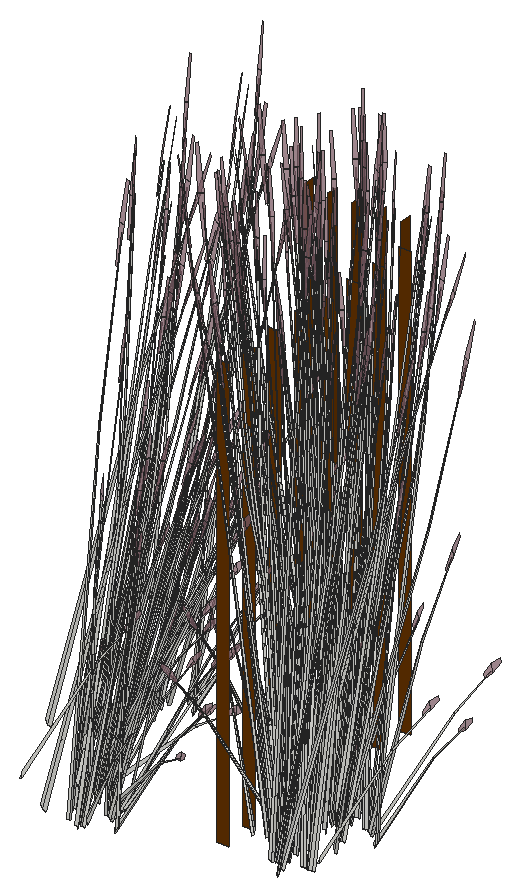
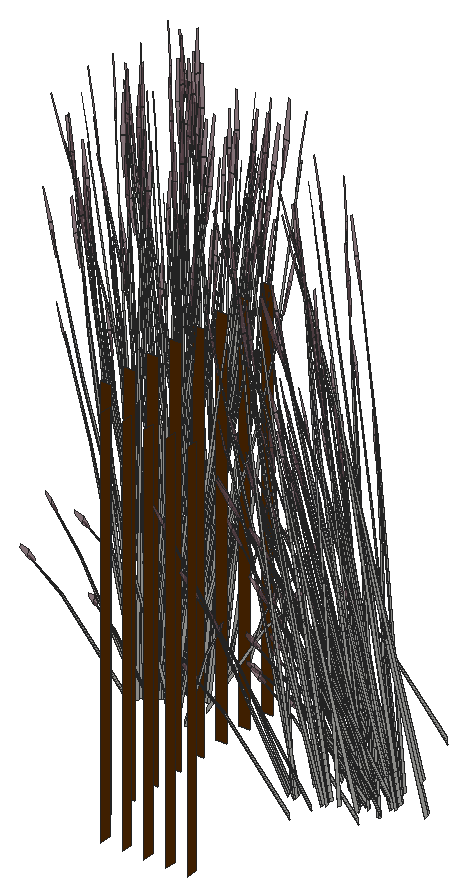
# SketchUp Ruby script. Lengths in inches.
U = 1.inch
M = Sketchup.active_model
def pt(a) = Geom::Point3d.new(a.map { |v| v * U })
def face(e, loops, mat)
  f = e.add_face(loops[0].map { |a| pt(a) })
  loops[1..].each { |l| e.add_face(l.map { |a| pt(a) }).erase! }
  f.material = f.back_material = mat if mat
  f
end
# faces: each face lists its corners as indices into pts; further lists are holes
def faces(e, pts, list, mat = nil) = list.each { |f| face(e, (f[0].is_a?(Array) ? f : [f]).map { |l| l.map { |i| pts[i] } }, mat) }
# xy, xz, yz: faces in a plane at the given z, y or x. An outline is a flat list of corners, or four numbers for a rectangle; further outlines are holes
def ring(l) = l.size == 4 ? [[l[0], l[1]], [l[2], l[1]], [l[2], l[3]], [l[0], l[3]]] : l.each_slice(2).to_a
def flat(e, list, mat, &to3) = list.each { |f| face(e, (f[0].is_a?(Array) ? f : [f]).map { |l| ring(l).map { |u, v| to3.(u, v) } }, mat) }
def xy(e, z, list, mat = nil) = flat(e, list, mat) { |x, y| [x, y, z] }
def xz(e, y, list, mat = nil) = flat(e, list, mat) { |x, z| [x, y, z] }
def yz(e, x, list, mat = nil) = flat(e, list, mat) { |y, z| [x, y, z] }
def lines(e, pts, list) = list.each { |a, b| e.add_line(pt(pts[a]), pt(pts[b])) }
# prism: a flat outline (further loops are holes) pulled along v
def prism(e, loops, v, mat = nil)
  f = face(e, loops, mat); d = Geom::Vector3d.new(v.map { |x| x * U })
  f.pushpull(f.normal.samedirection?(d) ? d.length : -d.length)
end
def box(e, o, s, mat = nil) = prism(e, [[o, [o[0] + s[0], o[1], o[2]], [o[0] + s[0], o[1] + s[1], o[2]], [o[0], o[1] + s[1], o[2]]]], [0, 0, s[2]], mat)
def at(x, y, z, deg = 0) = Geom::Transformation.translation(pt([x, y, z])) * Geom::Transformation.rotation(ORIGIN, Z_AXIS, deg.degrees)
def axes(o, x, y, z) = Geom::Transformation.new([*x, 0, *y, 0, *z, 0, *pt(o).to_a, 1])
def part(name) = M.definitions.add(name)
# library, detail: a bought-in or finely detailed component or shape, given as its bounding box
def library(name, o, s) = part(name).tap { |d| box(d.entities, o, s) }
def detail(e, o, s) = box(e.add_group.entities, o, s)
def put(e, d, t, mat = nil) = e.add_instance(d, t).tap { |i| i.material = mat if mat }
def group(e, t, mat = nil) = e.add_group.tap { |g| g.transformation = t; g.material = mat if mat }.entities
root = M.entities
M.materials.add("C08_Toffee_Ember").color = [102, 51, 0]
M.materials.add("LightPink_Translucent").color = [144, 107, 117]
M.materials["LightPink_Translucent"].alpha = 0.75
c1 = part("blade")
p = [[2.15,0.21,22],[0,0.17,0],[0.09,0.45,0],[2.18,0.31,22],[2.29,0.31,22],[0.38,0.45,0],
  [2.48,0.24,33],[2.49,0.24,33],[2.48,0.22,33]]
faces(c1.entities,p,[[0,1,2,3],[4,5,2,3],[6,3,4,7],[8,0,3,6]])
c2 = part("seeds")
p = [[0.3,-0.1,1.38],[-0.01,-0.03,1.59],[-0.01,-0.03,0.03],[0.14,-0.07,-0.07],[0.29,-0.03,3],[0.15,0.01,3.11]]
faces(c2.entities,p,[[0,1,2,3],[1,0,4,5]],"LightPink_Translucent")
c3 = part("blade with seeds")
put(c3.entities,c1,at(0,0,0))
put(c3.entities,c2,axes([2.4,0.25,30.99],[1.5799,-0.05474,1.17369],[-0.12525,1.92788,0.29478],[-0.07173,-0.02425,1.56792]))
xz(root,338.4,[[693.41,510,694.41,546]],"C08_Toffee_Ember")
xz(root,341.1,[[693.41,510,694.41,546]],"C08_Toffee_Ember")
xz(root,343.8,[[693.41,510,694.41,546]],"C08_Toffee_Ember")
xz(root,346.5,[[693.41,510,694.41,546]],"C08_Toffee_Ember")
xz(root,349.2,[[693.41,510,694.41,546]],"C08_Toffee_Ember")
xz(root,351.9,[[693.41,510,694.41,546]],"C08_Toffee_Ember")
xz(root,354.6,[[693.41,510,694.41,546]],"C08_Toffee_Ember")
xz(root,357.3,[[693.41,510,694.41,546]],"C08_Toffee_Ember")
yz(root,683.33,[[360,510,361,546]],"C08_Toffee_Ember")
yz(root,685.34,[[360,510,361,546]],"C08_Toffee_Ember")
yz(root,687.36,[[360,510,361,546]],"C08_Toffee_Ember")
yz(root,689.38,[[360,510,361,546]],"C08_Toffee_Ember")
yz(root,691.4,[[360,510,361,546]],"C08_Toffee_Ember")
put(root,c3,axes([681.33,342.92,511.97],[0.81352,0,0],[0,0.63814,-0.42834],[0,0.14534,1.3588]))
put(root,c3,axes([682.51,340.18,507.48],[0,-0.57097,0.4121],[0.72788,0,0],[0,0.13004,1.30728]))
put(root,c3,axes([678.7,342.09,512.21],[0.65687,-0.37907,-0.24149],[0.43681,0.53562,-0.41502],[0.16207,0.0544,1.32557]))
put(root,c3,axes([682.82,340.71,507.1],[0,0.57097,-0.4121],[-0.72788,0,0],[0,0.13004,1.30728]))
put(root,c3,axes([680.88,342.4375,509.35],[-0.64708,0.13103,0.39842],[-0.1123,-0.514,0.32852],[0.15218,0.15149,0.82444]))
put(root,c3,axes([680.76,342.54,509.35],[-0.29569,0.36271,0.05337],[-0.42107,-0.21117,0.42015],[0.13613,0.11629,0.64067]))
put(root,c3,axes([680.01,341.34,508.64],[-0.14872,-0.18332,1.42242],[0.6872,-0.15433,0.11501],[0.15531,0.28779,0.60807]))
put(root,c3,axes([680.44,339.28,507.6],[0.12551,-0.50956,0.12018],[0.6132,0.08845,-0.34318],[0.1116,0.05232,1.05198]))
put(root,c3,axes([680.07,348.69,511.83],[0.39083,0.47924,-0.37133],[-0.59199,0.33747,0.17871],[0.12647,0.0593,1.19224]))
put(root,c3,axes([679.34,335.47,511.24],[0.0474,-0.08243,1.46364],[0.59674,-0.24277,-0.2236],[0.18092,0.12565,0.24931]))
put(root,c3,axes([681.3125,338.39,507.48],[-0.60889,-0.28548,0.4121],[0.36394,-0.51192,0],[0.13868,0.06502,1.30728]))
put(root,c3,axes([679.87,350.69,512.15],[0.01148,-0.18927,1.18691],[0.54864,-0.21141,-0.25526],[0.16937,0.22654,0.50747]))
put(root,c3,axes([679.22,348.01,511.71],[0.43821,-0.42916,-0.51753],[0.54436,0.38915,-0.13583],[0.1756,-0.10706,1.14236]))
put(root,c3,axes([680.78,341.375,507.24],[0.68303,-0.19373,-0.15934],[0.24001,0.55805,0.00007],[0.07539,-0.02141,1.44335]))
put(root,c3,axes([677.04,341.75,511.32],[-0.64037,0.22859,1.07011],[-0.20382,-0.65589,0.4158],[0.39323,0.01091,1.21713]))
put(root,c3,axes([680.67,342.12,509.62],[-0.10048,-0.4599,0.29394],[0.5744,-0.12144,-0.37948],[0.15428,0.13179,0.72609]))
put(root,c3,axes([681.14,347.625,511.68],[0.15283,0.49751,-0.25712],[-0.60696,0.14127,0.25712],[0.12236,0.05737,1.15348]))
put(root,c3,axes([682.28,349.25,511.97],[0.81352,0,0],[0,0.63814,-0.42834],[0,0.14534,1.3588]))
put(root,c3,axes([679.99,340.74,511.97],[0.40676,-0.57214,0],[0.68052,0.31907,-0.42834],[0.15499,0.07267,1.3588]))
put(root,c3,axes([680.79,339.72,507.26],[0.39083,0.47924,-0.37133],[-0.59199,0.33747,0.17871],[0.12647,0.0593,1.19224]))
put(root,c3,axes([680.67,340.49,511.24],[-0.09738,-0.04498,1.46364],[-0.25012,-0.50252,-0.2236],[0.16873,-0.13637,0.24931]))
put(root,c3,axes([679.65,348.42,512.21],[0.65687,-0.37907,-0.24149],[0.43681,0.53562,-0.41502],[0.16207,0.0544,1.32557]))
put(root,c3,axes([681.05,339.48,509.14],[-0.56218,-0.29666,1.14775],[0.59361,-0.46189,0.49522],[0.18138,0.27836,1.10941]))
put(root,c3,axes([680.36,341.08,511.67],[0.60889,0.28548,-0.4121],[-0.36394,0.51192,0],[0.13868,0.06502,1.30728]))
put(root,c3,axes([680.11,342.77,509.33],[0.00193,-0.06913,1.47228],[0.55753,-0.30498,-0.13912],[0.19366,0.10886,0.26054]))
put(root,c3,axes([681.9,341.89,507.72],[-0.36631,-0.16417,0.95334],[0.47299,-0.16681,0.70045],[0.12758,0.1413,0.20998]))
put(root,c3,axes([680.6,341.72,507.57],[0.01148,-0.18927,1.18691],[0.54864,-0.21141,-0.25526],[0.16937,0.22654,0.50747]))
put(root,c3,axes([680.33,345.14,511.24],[0.0474,-0.08243,1.46364],[0.59674,-0.24277,-0.2236],[0.18092,0.12565,0.24931]))
put(root,c3,axes([679.47,342.17,511.71],[0.67676,0.09361,-0.51753],[-0.14281,0.57742,-0.13583],[0.20196,0.06997,1.14236]))
put(root,c3,axes([682.35,342.52,511.875],[-0.40335,-0.3651,-0.05385],[0.44175,-0.33453,-0.24415],[0.12517,-0.02355,0.8053]))
put(root,c3,axes([677.99,348.08,511.32],[-0.64037,0.22859,1.07011],[-0.20382,-0.65589,0.4158],[0.39323,0.01091,1.21713]))
put(root,c3,axes([681.86,338.65,507.11],[0.15283,0.49751,-0.25712],[-0.60696,0.14127,0.25712],[0.12236,0.05737,1.15348]))
put(root,c3,axes([683.01,340.28,507.4],[0.81352,0,0],[0,0.63814,-0.42834],[0,0.14534,1.3588]))
put(root,c3,axes([680.38,339.45,507.64],[0.65687,-0.37907,-0.24149],[0.43681,0.53562,-0.41502],[0.16207,0.0544,1.32557]))
put(root,c3,axes([681.96,342.64,507.64],[-0.4172,-0.01791,0.872],[0.27552,-0.38032,0.48145],[0.16481,0.13512,0.68401]))
put(root,c3,axes([682.33,339.38,509.62],[-0.56631,0.0816,0.29394],[-0.14954,-0.46647,-0.37948],[0.16229,-0.12529,0.72609]))
put(root,c3,axes([680.9375,347.07,511.97],[0.40676,-0.57214,0],[0.68052,0.31907,-0.42834],[0.15499,0.07267,1.3588]))
put(root,c3,axes([681.62,346.82,511.24],[-0.09738,-0.04498,1.46364],[-0.25012,-0.50252,-0.2236],[0.16873,-0.13637,0.24931]))
put(root,c3,axes([681.31,347.41,511.67],[0.60889,0.28548,-0.4121],[-0.36394,0.51192,0],[0.13868,0.06502,1.30728]))
put(root,c3,axes([681.28,351.47,511.24],[0.0474,-0.08243,1.46364],[0.59674,-0.24277,-0.2236],[0.18092,0.12565,0.24931]))
put(root,c3,axes([680.61,342.36,509.6],[0.38768,-0.48872,-0.10093],[0.56143,0.28156,-0.56021],[0.19516,0.13808,0.85122]))
put(root,c3,axes([678.72,339.11,506.75],[-0.64037,0.22859,1.07011],[-0.20382,-0.65589,0.4158],[0.39323,0.01091,1.21713]))
put(root,c3,axes([680.42,348.51,511.71],[0.67676,0.09361,-0.51753],[-0.14281,0.57742,-0.13583],[0.20196,0.06997,1.14236]))
put(root,c3,axes([683.3,348.85,511.875],[-0.40335,-0.3651,-0.05385],[0.44175,-0.33453,-0.24415],[0.12517,-0.02355,0.8053]))
put(root,c3,axes([681.07,342.12,509.31],[0.64198,-0.13573,-0.42412],[0.1123,0.514,-0.32852],[0.17243,0.1473,0.81151]))
put(root,c3,axes([681.66,338.1,507.4],[0.40676,-0.57214,0],[0.68052,0.31907,-0.42834],[0.15499,0.07267,1.3588]))
put(root,c3,axes([681.81,341.5,509.62],[-0.37017,-0.35748,0.29394],[0.42268,-0.3384,-0.37948],[0.21476,0.05149,0.72609]))
put(root,c3,axes([682.03,338.44,507.1],[0.60889,0.28548,-0.4121],[-0.36394,0.51192,0],[0.13868,0.06502,1.30728]))
put(root,c3,axes([682.15,341.83,509.35],[-0.03276,0.43418,0.05337],[-0.49468,-0.0119,0.42015],[0.18949,0.04543,0.64067]))
put(root,c3,axes([682,342.5,506.66],[0.0474,-0.08243,1.46364],[0.59674,-0.24277,-0.2236],[0.18092,0.12565,0.24931]))
put(root,c3,axes([682.19,341.6875,509.35],[-0.47971,0.37622,0.39842],[-0.41372,-0.39954,0.32852],[0.22506,0.0694,0.82444]))
put(root,c3,axes([683.4375,341.74,508.69],[-0.12452,-0.47997,-0.02898],[0.58854,-0.11034,-0.1314],[0.1229,0.03043,0.43341]))
put(root,c3,axes([682.42,340.5,509.62],[-0.54068,-0.15928,0.29394],[0.1577,-0.46469,-0.37948],[0.21769,-0.04261,0.72609]))
put(root,c3,axes([681.15,339.53,507.13],[0.67676,0.09361,-0.51753],[-0.14281,0.57742,-0.13583],[0.20196,0.06997,1.14236]))
put(root,c3,axes([684.03,339.875,507.3],[-0.40335,-0.3651,-0.05385],[0.44175,-0.33453,-0.24415],[0.12517,-0.02355,0.8053]))
put(root,c3,axes([681.16,341.49,512.15],[-0.23242,-0.01691,1.18691],[-0.23811,-0.45367,-0.25526],[0.28553,-0.12834,0.50747]))
put(root,c3,axes([683.1,338.02,507.72],[-0.2167,0.29065,0.95334],[-0.18626,-0.3905,0.70045],[0.17898,-0.09785,0.20998]))
put(root,c3,axes([682.84,339.31,509.35],[0.44663,0.24013,0.05337],[-0.26003,0.34195,0.42015],[0.14319,-0.11055,0.64067]))
put(root,c3,axes([682.72,339.21,509.35],[0.16135,0.52549,0.39842],[-0.63294,0.0912,0.32852],[0.18654,-0.12359,0.82444]))
put(root,c3,axes([681.59,343,511.65],[-0.41902,0.06852,1.17514],[-0.0667,-0.54541,0.06726],[0.29348,-0.08255,0.6687]))
put(root,c3,axes([682.04,342.64,511.24],[-0.034,-0.08668,1.46364],[0.23582,-0.50706,-0.2236],[0.23788,-0.00729,0.24931]))
put(root,c3,axes([681.01,340.77,508.64],[-0.24166,-0.09837,1.42242],[0.50011,-0.41269,0.11501],[0.3117,0.18617,0.60807]))
put(root,c3,axes([682.79,339.11,509.18],[0.56631,-0.0816,-0.29394],[0.14954,0.46647,0.37948],[0.16229,-0.12529,0.72609]))
put(root,c3,axes([682.91,340.64,509.35],[0.23895,0.38931,0.05337],[-0.43573,0.19055,0.42015],[0.19208,-0.0376,0.64067]))
put(root,c3,axes([682.33,341.6875,509.18],[0.37017,0.35748,-0.29394],[-0.42268,0.3384,0.37948],[0.21476,0.05149,0.72609]))
put(root,c3,axes([681.91,341.73,509.6],[0.03484,-0.58066,-0.10093],[0.65957,0.01587,-0.56021],[0.25402,0.04034,0.85122]))
put(root,c3,axes([682.65,340.65,509.6],[-0.32734,-0.51701,-0.10093],[0.58097,-0.25407,-0.56021],[0.24483,-0.06821,0.85122]))
put(root,c3,axes([682.86,340.51,509.35],[-0.18381,0.5206,0.39842],[-0.60429,-0.17802,0.32852],[0.23764,-0.03129,0.82444]))
put(root,c3,axes([682.11,347.82,512.15],[-0.23242,-0.01691,1.18691],[-0.23811,-0.45367,-0.25526],[0.28553,-0.12834,0.50747]))
put(root,c3,axes([682.54,349.33,511.65],[-0.41902,0.06852,1.17514],[-0.0667,-0.54541,0.06726],[0.29348,-0.08255,0.6687]))
put(root,c3,axes([682.48,341.38,509.34],[0.13956,-0.00966,1.45204],[0.38281,-0.44358,-0.22964],[0.24825,0.05855,0.11645]))
put(root,c3,axes([681.71,343.81,512.15],[-0.15668,-0.14043,1.18691],[0.20386,-0.46454,-0.25526],[0.31701,0.06293,0.50747]))
put(root,c3,axes([683,348.97,511.24],[-0.034,-0.08668,1.46364],[0.23582,-0.50706,-0.2236],[0.23788,-0.00729,0.24931]))
put(root,c3,axes([682.62,340.21,509.31],[0.17625,-0.51936,-0.42412],[0.60429,0.17802,-0.32852],[0.2433,-0.04762,0.81151]))
put(root,c3,axes([684.14,340.54,507.72],[-0.40197,0.09426,0.95334],[0.18921,-0.38956,0.70045],[0.21325,0.02666,0.20998]))
put(root,c3,axes([682.99,340.45,509.18],[0.54068,0.15928,-0.29394],[-0.1577,0.46469,0.37948],[0.21769,-0.04261,0.72609]))
put(root,c3,axes([681.94,341.45,509.56],[0.65035,0.01375,-0.58968],[-0.04368,0.5789,0.07116],[0.27552,0.06109,0.83415]))
put(root,c3,axes([683.26,340.36,507.07],[-0.41902,0.06852,1.17514],[-0.0667,-0.54541,0.06726],[0.29348,-0.08255,0.6687]))
put(root,c3,axes([683.72,340,506.66],[-0.034,-0.08668,1.46364],[0.23582,-0.50706,-0.2236],[0.23788,-0.00729,0.24931]))
put(root,c3,axes([683.95,342.19,509.33],[-0.05883,-0.04999,1.47228],[0.12868,-0.53581,-0.13912],[0.23172,-0.03423,0.26054]))
put(root,c3,axes([681.52,339.87,508.64],[-0.26985,0.01293,1.42242],[0.17902,-0.56047,0.11501],[0.38456,0.03467,0.60807]))
put(root,c3,axes([682.66,350.14,512.15],[-0.15668,-0.14043,1.18691],[0.20386,-0.46454,-0.25526],[0.31701,0.06293,0.50747]))
put(root,c3,axes([682.5,340.4,509.56],[0.57168,-0.25217,-0.58968],[0.3186,0.51908,0.07116],[0.27622,-0.05897,0.83415]))
put(root,c3,axes([684.42,339.84,509.34],[0.09028,-0.08697,1.45204],[-0.11555,-0.53348,-0.22964],[0.22652,-0.10115,0.11645]))
put(root,c3,axes([683.38,341.17,507.57],[-0.15668,-0.14043,1.18691],[0.20386,-0.46454,-0.25526],[0.31701,0.06293,0.50747]))
put(root,c3,axes([696.2,342.55,511.24],[0.0165,0.08998,1.46364],[-0.33262,0.46992,-0.2236],[-0.23626,-0.02369,0.24931]))
put(root,c3,axes([696.02,338.67,511.24],[0.08727,0.05704,1.46364],[0.14797,0.52853,-0.2236],[-0.19341,0.11271,0.24931]))
put(root,c3,axes([696.02,345.07,511.24],[0.08727,0.05704,1.46364],[0.14797,0.52853,-0.2236],[-0.19341,0.11271,0.24931]))
put(root,c3,axes([698.37,343.37,511.71],[-0.67676,-0.09361,-0.51753],[0.14281,-0.57742,-0.13583],[-0.20196,-0.06997,1.14236]))
put(root,c3,axes([697.48,344.46,511.67],[-0.60889,-0.28548,-0.4121],[0.36394,-0.51192,0],[-0.13868,-0.06502,1.30728]))
put(root,c3,axes([697.22,340.21,511.24],[-0.06302,0.07522,1.46364],[-0.63686,0.16217,-0.2236],[-0.15385,-0.14752,0.24931]))
put(root,c3,axes([697.86,338.41,511.97],[-0.40676,0.57214,0],[-0.68052,-0.31907,-0.42834],[-0.15499,-0.07267,1.3588]))
put(root,c3,axes([697.86,344.81,511.97],[-0.40676,0.57214,0],[-0.68052,-0.31907,-0.42834],[-0.15499,-0.07267,1.3588]))
put(root,c3,axes([696.82,340.5,511.77],[-0.18768,0.46622,-0.03231],[-0.57763,-0.14342,-0.14649],[-0.0877,-0.07626,0.48318]))
put(root,c3,axes([699.14,343.45,512.21],[-0.65687,0.37907,-0.24149],[-0.43681,-0.53562,-0.41502],[-0.16207,-0.0544,1.32557]))
put(root,c3,axes([696.51,342.63,511.97],[-0.81352,0,0],[0,-0.63814,-0.42834],[0,-0.14534,1.3588]))
put(root,c3,axes([697.65,344.25,511.68],[-0.15283,-0.49751,-0.25712],[0.60696,-0.14127,0.25712],[-0.12236,-0.05737,1.15348]))
put(root,c3,axes([699.58,337.47,511.71],[-0.43821,0.42916,-0.51753],[-0.54436,-0.38915,-0.13583],[-0.1756,0.10706,1.14236]))
put(root,c3,axes([699.58,343.87,511.71],[-0.43821,0.42916,-0.51753],[-0.54436,-0.38915,-0.13583],[-0.1756,0.10706,1.14236]))
put(root,c3,axes([697.14,342.46,511.93],[-0.60515,0.48003,0.25528],[-0.60552,-0.47498,-0.30288],[-0.02113,-0.13632,1.36855]))
put(root,c3,axes([699.88,337.23,512.05],[-0.63528,-0.45956,-0.20909],[0.53456,-0.51604,0.45758],[-0.17107,0.05376,1.39619]))
put(root,c3,axes([699.88,343.63,512.05],[-0.63528,-0.45956,-0.20909],[0.53456,-0.51604,0.45758],[-0.17107,0.05376,1.39619]))
put(root,c3,axes([698.72,343.19,511.83],[-0.39083,-0.47924,-0.37133],[0.59199,-0.33747,0.17871],[-0.12647,-0.0593,1.19224]))
put(root,c3,axes([699.56,337.13,511.83],[-0.70648,0.03525,-0.37133],[-0.06389,-0.58508,0.17871],[-0.12647,0.0593,1.19224]))
put(root,c3,axes([699.56,343.53,511.83],[-0.70648,0.03525,-0.37133],[-0.06389,-0.58508,0.17871],[-0.12647,0.0593,1.19224]))
put(root,c3,axes([698.78,343.46,512.02],[0.17244,-0.67657,-0.19446],[0.81759,0.11793,0.42555],[-0.14286,-0.09343,1.29846]))
put(root,c3,axes([699.08,337.22,512.17],[-0.12551,0.50956,0.12018],[-0.6132,-0.08845,-0.34318],[-0.1116,-0.05232,1.05198]))
put(root,c3,axes([699.08,343.62,512.17],[-0.12551,0.50956,0.12018],[-0.6132,-0.08845,-0.34318],[-0.1116,-0.05232,1.05198]))
put(root,c3,axes([700.3,338.64,511.67],[-0.60889,0.28548,-0.4121],[-0.36394,-0.51192,0],[-0.13868,0.06502,1.30728]))
put(root,c3,axes([700.3,345.04,511.67],[-0.60889,0.28548,-0.4121],[-0.36394,-0.51192,0],[-0.13868,0.06502,1.30728]))
put(root,c3,axes([696.69,342.19,511.67],[0,-0.57097,-0.4121],[0.72788,0,0],[0,-0.13004,1.30728]))
put(root,c3,axes([700.34,338.49,511.82],[-0.40169,-0.57414,-0.04268],[0.68052,-0.31907,0.42834],[-0.16769,0.05466,1.35813]))
put(root,c3,axes([700.34,344.89,511.82],[-0.40169,-0.57414,-0.04268],[0.68052,-0.31907,0.42834],[-0.16769,0.05466,1.35813]))
put(root,c3,axes([700.16,338.41,511.68],[-0.60696,-0.14127,-0.25712],[0.15283,-0.49751,0.25712],[-0.12236,0.05737,1.15348]))
put(root,c3,axes([700.16,344.8125,511.68],[-0.60696,-0.14127,-0.25712],[0.15283,-0.49751,0.25712],[-0.12236,0.05737,1.15348]))
put(root,c3,axes([698.6,342.86,512.21],[-0.73268,-0.27244,-0.24149],[0.35279,-0.57501,-0.41502],[-0.02303,-0.14118,1.32557]))
put(root,c3,axes([697.26,338.8,512.34],[0.59102,-0.10111,0.05401],[0.13587,0.40735,-0.71633],[-0.03747,0.2062,0.64209]))
put(root,c3,axes([697.26,345.2,512.34],[0.59102,-0.10111,0.05401],[0.13587,0.40735,-0.71633],[-0.03747,0.2062,0.64209]))
put(root,c3,axes([700.05,336.97,512.21],[0.07581,0.65151,-0.24149],[-0.7896,0.03939,-0.41502],[-0.13904,0.08678,1.32557]))
put(root,c3,axes([700.05,343.37,512.21],[0.07581,0.65151,-0.24149],[-0.7896,0.03939,-0.41502],[-0.13904,0.08678,1.32557]))
put(root,c3,axes([698.27,342.28,511.74],[-0.26718,-0.5855,-0.57963],[0.76964,-0.21087,-0.15213],[-0.02953,-0.19827,1.27944]))
put(root,c3,axes([697.01,342.21,511.68],[0.45414,-0.35624,-0.25712],[0.45414,0.35624,0.25712],[0,-0.11474,1.15348]))
put(root,c3,axes([699.06,339.9,511.77],[-0.44958,0.32756,-0.03231],[-0.41194,-0.35875,-0.14649],[-0.029,-0.10165,0.48318]))
put(root,c3,axes([698.875,343.13,511.96],[0.82229,0.1203,0.37976],[-0.16734,0.67942,0.14902],[-0.12017,-0.06561,1.31851]))
put(root,c3,axes([699.33,337.91,511.82],[-0.65588,-0.25634,0],[0.31565,-0.53263,0],[0,0,1.35047]))
put(root,c3,axes([699.33,344.31,511.82],[-0.65588,-0.25634,0],[0.31565,-0.53263,0],[0,0,1.35047]))
put(root,c3,axes([700.85,338.55,511.97],[0.40676,0.57214,0],[-0.68052,0.31907,-0.42834],[-0.15499,0.07267,1.3588]))
put(root,c3,axes([700.85,344.95,511.97],[0.40676,0.57214,0],[-0.68052,0.31907,-0.42834],[-0.15499,0.07267,1.3588]))
put(root,c3,axes([700.2,337.1,512.17],[0.48065,0.34305,0.12018],[-0.40092,0.38703,-0.34318],[-0.1116,0.05232,1.05198]))
put(root,c3,axes([700.2,343.5,512.17],[0.48065,0.34305,0.12018],[-0.40092,0.38703,-0.34318],[-0.1116,0.05232,1.05198]))
put(root,c3,axes([700.03,343.07,511.91],[-0.60515,-0.49144,-0.05089],[0.60552,-0.49174,0],[-0.02113,-0.01716,1.45724]))
put(root,c3,axes([700.36,338.19,511.93],[0.81449,0.18558,0.25528],[-0.20377,0.66335,-0.30288],[-0.13481,0.08302,1.36855]))
put(root,c3,axes([700.36,344.59,511.93],[0.81449,0.18558,0.25528],[-0.20377,0.66335,-0.30288],[-0.13481,0.08302,1.36855]))
put(root,c3,axes([698.8,342.51,511.96],[0.28286,0.63846,0.37976],[-0.80821,0.22202,0.14902],[0.00988,-0.11732,1.31851]))
put(root,c3,axes([698.67,342.43,511.83],[0.31565,-0.51449,-0.37133],[0.65588,0.24761,0.17871],[0,-0.1186,1.19224]))
put(root,c3,axes([699.48,337.6875,511.83],[-0.21227,-0.49226,0],[0.60616,-0.17239,0],[0,0,1.28128]))
put(root,c3,axes([699.48,344.09,511.83],[-0.21227,-0.49226,0],[0.60616,-0.17239,0],[0,0,1.28128]))
put(root,c3,axes([698.71,338.73,511.24],[0.10529,-0.03107,1.46364],[0.63335,0.17101,-0.2236],[0.01852,0.19274,0.24931]))
put(root,c3,axes([698.71,345.125,511.24],[0.10529,-0.03107,1.46364],[0.63335,0.17101,-0.2236],[0.01852,0.19274,0.24931]))
put(root,c3,axes([700.34,336.72,511.83],[-0.31565,0.51449,-0.37133],[-0.65588,-0.24761,0.17871],[0,0.1186,1.19224]))
put(root,c3,axes([700.34,343.12,511.83],[-0.31565,0.51449,-0.37133],[-0.65588,-0.24761,0.17871],[0,0.1186,1.19224]))
put(root,c3,axes([699.82,342.5625,511.83],[0,-0.66065,0],[0.81352,0,0],[0,0,1.48949]))
put(root,c3,axes([699.07,342.68,512.02],[0.73304,0.27674,0.19974],[-0.35279,0.57501,0.41502],[0,-0.13255,1.3325]))
put(root,c3,axes([700.23,336.43,511.9],[0,0.66033,-0.04679],[-0.81352,0,0],[0,0.02075,1.48875]))
put(root,c3,axes([700.23,342.83,511.9],[0,0.66033,-0.04679],[-0.81352,0,0],[0,0.02075,1.48875]))
put(root,c3,axes([699.84,337.7,511.9],[0.28286,0.65594,-0.0499],[-0.80821,0.22985,0],[0.00988,0.02291,1.42904]))
put(root,c3,axes([699.84,344.1,511.9],[0.28286,0.65594,-0.0499],[-0.80821,0.22985,0],[0.00988,0.02291,1.42904]))
put(root,c3,axes([698.16,340.59,511.97],[-0.40676,-0.57214,0],[0.68052,-0.31907,-0.42834],[0.15499,-0.07267,1.3588]))
put(root,c3,axes([702.18,336.84,511.83],[-0.81312,-0.00457,-0.0413],[0,-0.63814,0.41452],[-0.02555,0.14527,1.31432]))
put(root,c3,axes([702.18,343.24,511.83],[-0.81312,-0.00457,-0.0413],[0,-0.63814,0.41452],[-0.02555,0.14527,1.31432]))
put(root,c3,axes([699.4375,342.15,511.96],[-0.53943,0.51816,0.37976],[-0.64086,-0.4574,0.14902],[0.13005,-0.05171,1.31851]))
put(root,c3,axes([700.36,336.5625,511.84],[0.45414,0.3688,0],[-0.45414,0.3688,0],[0,0,1.40491]))
put(root,c3,axes([700.36,342.96,511.84],[0.45414,0.3688,0],[-0.45414,0.3688,0],[0,0,1.40491]))
put(root,c3,axes([700.08,337.92,511.83],[0.65588,0.25634,0],[-0.31565,0.53263,0],[0,0,1.45212]))
put(root,c3,axes([700.08,344.32,511.83],[0.65588,0.25634,0],[-0.31565,0.53263,0],[0,0,1.45212]))
put(root,c3,axes([700.14,336.01,511.98],[-0.82229,-0.1203,0.40835],[0.16734,-0.67942,0.16024],[0.12017,0.06561,1.41775]))
put(root,c3,axes([700.14,342.41,511.98],[-0.82229,-0.1203,0.40835],[0.16734,-0.67942,0.16024],[0.12017,0.06561,1.41775]))
put(root,c3,axes([702.01,336.9375,511.68],[-0.45414,0.35624,-0.25712],[-0.45414,-0.35624,0.25712],[0,0.11474,1.15348]))
put(root,c3,axes([702.01,343.34,511.68],[-0.45414,0.35624,-0.25712],[-0.45414,-0.35624,0.25712],[0,0.11474,1.15348]))
put(root,c3,axes([700.71,336.87,511.74],[0.23855,0.52277,-0.57446],[-0.68718,0.18827,-0.15077],[0.02637,0.17702,1.26801]))
put(root,c3,axes([700.71,343.27,511.74],[0.23855,0.52277,-0.57446],[-0.68718,0.18827,-0.15077],[0.02637,0.17702,1.26801]))
put(root,c3,axes([700.375,342.71,511.83],[0.72788,0,0],[0,0.59111,0],[0,0,1.48078]))
put(root,c3,axes([698.96,342.17,512.21],[-0.07581,-0.65151,-0.24149],[0.7896,-0.03939,-0.41502],[0.13904,-0.08678,1.32557]))
put(root,c3,axes([700.625,336.25,512.17],[0.60616,-0.16651,0.12018],[0.21227,0.47548,-0.34318],[0,0.10465,1.05198]))
put(root,c3,axes([700.625,342.65,512.17],[0.60616,-0.16651,0.12018],[0.21227,0.47548,-0.34318],[0,0.10465,1.05198]))
put(root,c3,axes([700.42,336.29,512.21],[0.73268,0.27244,-0.24149],[-0.35279,0.57501,-0.41502],[0.02303,0.14118,1.32557]))
put(root,c3,axes([700.42,342.6875,512.21],[0.73268,0.27244,-0.24149],[-0.35279,0.57501,-0.41502],[0.02303,0.14118,1.32557]))
put(root,c3,axes([698.86,340.73,511.68],[0.60696,0.14127,-0.25712],[-0.15283,0.49751,0.25712],[0.12236,-0.05737,1.15348]))
put(root,c3,axes([702.32,336.95,511.67],[0,0.57097,-0.4121],[-0.72788,0,0],[0,0.13004,1.30728]))
put(root,c3,axes([702.32,343.35,511.67],[0,0.57097,-0.4121],[-0.72788,0,0],[0,0.13004,1.30728]))
put(root,c3,axes([698.72,340.5,511.67],[0.60889,-0.28548,-0.4121],[0.36394,0.51192,0],[0.13868,-0.06502,1.30728]))
put(root,c3,axes([699.9375,341.92,512.17],[0.12551,-0.50956,0.12018],[0.6132,0.08845,-0.34318],[0.1116,0.05232,1.05198]))
put(root,c3,axes([700.28,337.62,511.8125],[0.68303,-0.19373,-0.15934],[0.24001,0.55805,0.00007],[0.07539,-0.02141,1.44335]))
put(root,c3,axes([700.28,344.02,511.8125],[0.68303,-0.19373,-0.15934],[0.24001,0.55805,0.00007],[0.07539,-0.02141,1.44335]))
put(root,c3,axes([700.29,335.96,511.83],[0.39083,0.47924,-0.37133],[-0.59199,0.33747,0.17871],[0.12647,0.0593,1.19224]))
put(root,c3,axes([700.29,342.36,511.83],[0.39083,0.47924,-0.37133],[-0.59199,0.33747,0.17871],[0.12647,0.0593,1.19224]))
put(root,c3,axes([699.4375,341.68,511.71],[0.43821,-0.42916,-0.51753],[0.54436,0.38915,-0.13583],[0.1756,-0.10706,1.14236]))
put(root,c3,axes([701.36,334.89,511.68],[0.15283,0.49751,-0.25712],[-0.60696,0.14127,0.25712],[0.12236,0.05737,1.15348]))
put(root,c3,axes([701.36,341.29,511.68],[0.15283,0.49751,-0.25712],[-0.60696,0.14127,0.25712],[0.12236,0.05737,1.15348]))
put(root,c3,axes([702.5,336.52,511.97],[0.81352,0,0],[0,0.63814,-0.42834],[0,0.14534,1.3588]))
put(root,c3,axes([702.5,342.92,511.97],[0.81352,0,0],[0,0.63814,-0.42834],[0,0.14534,1.3588]))
put(root,c3,axes([699.875,342.09,512.21],[0.65687,-0.37907,-0.24149],[0.43681,0.53562,-0.41502],[0.16207,0.0544,1.32557]))
put(root,c3,axes([698.22,341.75,511.32],[-0.64037,0.22859,1.07011],[-0.20382,-0.65589,0.4158],[0.39323,0.01091,1.21713]))
put(root,c3,axes([701.16,340.74,511.97],[0.40676,-0.57214,0],[0.68052,0.31907,-0.42834],[0.15499,0.07267,1.3588]))
put(root,c3,axes([701.84,340.49,511.24],[-0.09738,-0.04498,1.46364],[-0.25012,-0.50252,-0.2236],[0.16873,-0.13637,0.24931]))
put(root,c3,axes([701.53,341.08,511.67],[0.60889,0.28548,-0.4121],[-0.36394,0.51192,0],[0.13868,0.06502,1.30728]))
put(root,c3,axes([701.5,338.74,511.24],[0.0474,-0.08243,1.46364],[0.59674,-0.24277,-0.2236],[0.18092,0.12565,0.24931]))
put(root,c3,axes([701.5,345.14,511.24],[0.0474,-0.08243,1.46364],[0.59674,-0.24277,-0.2236],[0.18092,0.12565,0.24931]))
put(root,c3,axes([700.64,335.77,511.71],[0.67676,0.09361,-0.51753],[-0.14281,0.57742,-0.13583],[0.20196,0.06997,1.14236]))
put(root,c3,axes([700.64,342.17,511.71],[0.67676,0.09361,-0.51753],[-0.14281,0.57742,-0.13583],[0.20196,0.06997,1.14236]))
put(root,c3,axes([703.52,342.52,511.875],[-0.40335,-0.3651,-0.05385],[0.44175,-0.33453,-0.24415],[0.12517,-0.02355,0.8053]))
put(root,c3,axes([702.76,343,511.65],[-0.41902,0.06852,1.17514],[-0.0667,-0.54541,0.06726],[0.29348,-0.08255,0.6687]))
put(root,c3,axes([703.22,342.64,511.24],[-0.034,-0.08668,1.46364],[0.23582,-0.50706,-0.2236],[0.23788,-0.00729,0.24931]))
